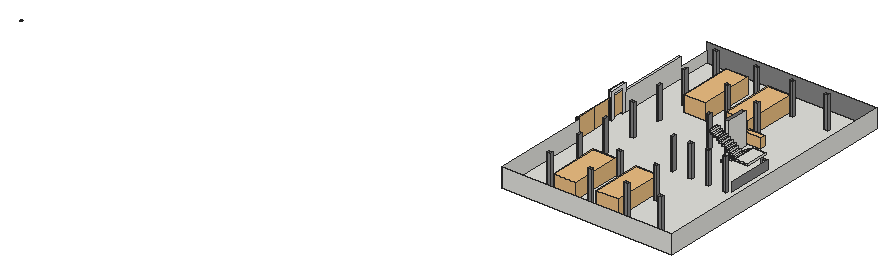
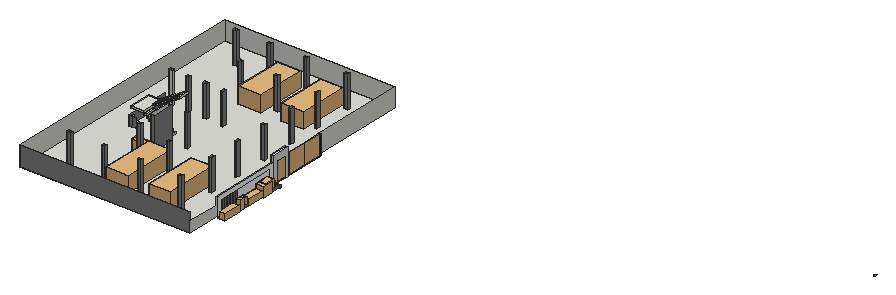
# SketchUp Ruby script. Lengths in inches.
U = 1.inch
M = Sketchup.active_model
def pt(a) = Geom::Point3d.new(a.map { |v| v * U })
def face(e, loops, mat)
  f = e.add_face(loops[0].map { |a| pt(a) })
  loops[1..].each { |l| e.add_face(l.map { |a| pt(a) }).erase! }
  f.material = f.back_material = mat if mat
  f
end
# faces: each face lists its corners as indices into pts; further lists are holes
def faces(e, pts, list, mat = nil) = list.each { |f| face(e, (f[0].is_a?(Array) ? f : [f]).map { |l| l.map { |i| pts[i] } }, mat) }
# xy, xz, yz: faces in a plane at the given z, y or x. An outline is a flat list of corners, or four numbers for a rectangle; further outlines are holes
def ring(l) = l.size == 4 ? [[l[0], l[1]], [l[2], l[1]], [l[2], l[3]], [l[0], l[3]]] : l.each_slice(2).to_a
def flat(e, list, mat, &to3) = list.each { |f| face(e, (f[0].is_a?(Array) ? f : [f]).map { |l| ring(l).map { |u, v| to3.(u, v) } }, mat) }
def xy(e, z, list, mat = nil) = flat(e, list, mat) { |x, y| [x, y, z] }
def xz(e, y, list, mat = nil) = flat(e, list, mat) { |x, z| [x, y, z] }
def yz(e, x, list, mat = nil) = flat(e, list, mat) { |y, z| [x, y, z] }
def lines(e, pts, list) = list.each { |a, b| e.add_line(pt(pts[a]), pt(pts[b])) }
# prism: a flat outline (further loops are holes) pulled along v
def prism(e, loops, v, mat = nil)
  f = face(e, loops, mat); d = Geom::Vector3d.new(v.map { |x| x * U })
  f.pushpull(f.normal.samedirection?(d) ? d.length : -d.length)
end
def box(e, o, s, mat = nil) = prism(e, [[o, [o[0] + s[0], o[1], o[2]], [o[0] + s[0], o[1] + s[1], o[2]], [o[0], o[1] + s[1], o[2]]]], [0, 0, s[2]], mat)
def at(x, y, z, deg = 0) = Geom::Transformation.translation(pt([x, y, z])) * Geom::Transformation.rotation(ORIGIN, Z_AXIS, deg.degrees)
def axes(o, x, y, z) = Geom::Transformation.new([*x, 0, *y, 0, *z, 0, *pt(o).to_a, 1])
def part(name) = M.definitions.add(name)
# library, detail: a bought-in or finely detailed component or shape, given as its bounding box
def library(name, o, s) = part(name).tap { |d| box(d.entities, o, s) }
def detail(e, o, s) = box(e.add_group.entities, o, s)
def put(e, d, t, mat = nil) = e.add_instance(d, t).tap { |i| i.material = mat if mat }
def group(e, t, mat = nil) = e.add_group.tap { |g| g.transformation = t; g.material = mat if mat }.entities
root = M.entities
M.materials.add("Bricks Weathered E01 100cm\#1").color = [154, 112, 93]
M.materials.add("Marble White 602 38.29cm").color = [255, 255, 255]
M.materials.add("Metal Black").color = [38, 38, 38]
M.materials.add("Mud Stones 01 100cm").color = [155, 124, 86]
M.materials.add("Paint Brown Gloss 1.5cm").color = [255, 255, 255]
M.materials.add("Wall Paint Bumpy 01 Gray 100cm").color = [135, 135, 135]
M.materials.add("Wood Planks C01 100cm\#1").color = [136, 107, 89]
M.materials.add("[Polished Concrete Old]").color = [229, 229, 229]
c1 = library("Comptonia peregrina 005",[-33.17,-28.03,-1.38],[76.14,61.63,51.11])
c2 = library("Potted Plant 02",[-16.98,-19.78,0],[30.04,38.68,37.52])
c3 = library("bike",[-29.48,-10.91,0],[58.96,21.79,36.68])
c4 = part("Rectangular post")
xy(c4.entities,0,[[0,0,2.7,4.37]])
xy(c4.entities,59.3,[[0,0,2.7,4.37]])
xz(c4.entities,0,[[0,0,2.7,59.3]])
xz(c4.entities,4.37,[[0,0,2.7,59.3]],"Wood Planks C01 100cm\#1")
yz(c4.entities,0,[[0,0,4.37,59.3]],"Wood Planks C01 100cm\#1")
yz(c4.entities,2.7,[[0,0,4.37,59.3]])
c5 = library("Group\#43",[0,0,0],[42,3,72])
c6 = library("Group\#38",[0.25,0,0],[71.75,3,72.2])
c7 = library("Group\#39",[0.25,0,0],[71.75,3,72.2])
c8 = part("Stair tread \#1")
box(c8.entities,[0,0,0],[10,39,7])
c9 = part("Stair tread")
box(c9.entities,[0,0,0],[10,39,7])
c10 = part("Group\#13")
box(c10.entities,[100,0,63],[49,84,7])
put(c10.entities,c8,at(50,45,28))
put(c10.entities,c8,at(20,45,7))
put(c10.entities,c8,at(90,45,56))
put(c10.entities,c8,at(70,45,42))
put(c10.entities,c8,at(40,45,21))
put(c10.entities,c8,at(60,45,35))
put(c10.entities,c8,at(10,45,0))
put(c10.entities,c8,at(30,45,14))
put(c10.entities,c8,at(80,45,49))
put(c10.entities,c9,at(90,0,70))
put(c10.entities,c9,at(10,0,126))
put(c10.entities,c9,at(60,0,91))
put(c10.entities,c9,at(30,0,112))
put(c10.entities,c9,at(50,0,98))
put(c10.entities,c9,at(70,0,84))
put(c10.entities,c9,at(80,0,77))
put(c10.entities,c9,at(40,0,105))
put(c10.entities,c9,at(0,0,133))
put(c10.entities,c9,at(20,0,119))
c11 = library("Car 038",[-41.0625,-100.42,-1.26],[82.125,200.85,59.95])
c12 = library("Group\#48",[0,0,0],[3.9375,4.89,0.01])
c13 = library("Group1671\#3",[0,0,0],[3.9375,4.89,0.39])
c14 = library("Group1672\#2",[0,0,0],[3.9375,4.89,0.39])
c15 = library("Car 033",[-43.24,-98.19,-1.29],[86.48,201.64,57.79])
c16 = library("Dalea purpurea 001",[-8.36,-8.34,-0.5],[17.08,16.6,23.28])
c17 = library("Car 026",[-43.02,-94.05,-1.1],[86.04,187.94,58.68])
c18 = library("Sedum Plant 66-24",[-7.97,-7.95,0.04],[16.42,16.31,19.57])
xy(root,0,[[[1741.02,413.67,2384.52,413.67,2384.52,1382.67,1741.02,1382.67,1741.02,1000.17,1729.02,1000.17,1729.02,778.17,1741.02,778.17],[2132.52,980.67,2146.52,1061.67],[1843.02,1286.67,1857.02,1295.67],[1843.02,500.67,1857.02,509.67],[2262.52,806.67,2276.52,815.67],[1843.02,641.67,1852.02,655.67],[1843.02,763.67,1852.02,777.67],[1843.02,1018.67,1852.02,1032.67],[1843.02,1140.67,1852.02,1154.67],[2066.52,806.67,2075.52,820.67],[2135.52,500.67,2149.52,509.67],[1997.02,638.67,2011.02,647.67],[2132.52,806.67,2146.52,815.67],[2066.52,975.67,2075.52,989.67],[1843.02,893.67,1857.02,902.67],[2132.52,1118.67,2146.52,1127.67],[1997.02,1148.67,2011.02,1157.67],[1997.02,1286.67,2011.02,1295.67],[1997.02,500.67,2011.02,509.67],[2262.52,500.67,2276.52,509.67],[2198.52,806.67,2212.52,815.67],[2262.52,1286.67,2276.52,1295.67],[2135.52,638.67,2149.52,647.67],[2132.52,1286.67,2146.52,1295.67]],[1843.02,500.67,1857.02,509.67],[1997.02,500.67,2011.02,509.67],[2135.52,500.67,2149.52,509.67],[2262.52,500.67,2276.52,509.67],
  [2132.52,989.67,2146.52,1061.67],[1843.02,1286.67,1857.02,1295.67],[1997.02,1286.67,2011.02,1295.67],[2132.52,1286.67,2146.52,1295.67],[2262.52,1286.67,2276.52,1295.67]])
xy(root,0,[[1709.32,1005.17,1733.02,1005.17,1733.02,1014.17,1740.02,1014.17,1740.02,1248.68,1733.02,1248.68,1733.02,1257.65,1709.32,1257.65]],"Mud Stones 01 100cm")
xy(root,0,[[1704.32,1000.17,1733.02,1001.07]],"Paint Brown Gloss 1.5cm")
xz(root,413.67,[[1741.02,0,2384.52,72]])
xz(root,500.67,[[1843.02,0,1857.02,120],[1997.02,0,2011.02,120],[2135.52,0,2149.52,120],[2262.52,0,2276.52,120]],"Wall Paint Bumpy 01 Gray 100cm")
xz(root,509.67,[[1843.02,0,1857.02,120],[1997.02,0,2011.02,120],[2135.52,0,2149.52,120],[2262.52,0,2276.52,120]],"Wall Paint Bumpy 01 Gray 100cm")
xz(root,638.67,[[1997.02,0,2011.02,120],[2135.52,0,2149.52,120]],"Wall Paint Bumpy 01 Gray 100cm")
xz(root,641.67,[[1843.02,0,1852.02,120]],"Wall Paint Bumpy 01 Gray 100cm")
xz(root,647.67,[[1997.02,0,2011.02,120],[2135.52,0,2149.52,120]],"Wall Paint Bumpy 01 Gray 100cm")
xz(root,655.67,[[1843.02,0,1852.02,120]],"Wall Paint Bumpy 01 Gray 100cm")
xz(root,763.67,[[1843.02,0,1852.02,120]],"Wall Paint Bumpy 01 Gray 100cm")
xz(root,777.67,[[1843.02,0,1852.02,120]],"Wall Paint Bumpy 01 Gray 100cm")
xz(root,778.17,[[1729.02,0,1741.02,72]])
xz(root,806.67,[[2066.52,0,2075.52,120],[2132.52,0,2146.52,120],[2198.52,0,2212.52,120],[2262.52,0,2276.52,120]],"Wall Paint Bumpy 01 Gray 100cm")
xz(root,815.67,[[2262.52,0,2276.52,120]])
xz(root,815.67,[[2132.52,0,2146.52,120],[2198.52,0,2212.52,120]],"Wall Paint Bumpy 01 Gray 100cm")
xz(root,820.67,[[2066.52,0,2075.52,120]],"Wall Paint Bumpy 01 Gray 100cm")
xz(root,893.67,[[1843.02,0,1857.02,120]],"Wall Paint Bumpy 01 Gray 100cm")
xz(root,902.67,[[1843.02,0,1857.02,120]],"Wall Paint Bumpy 01 Gray 100cm")
xz(root,975.67,[[2066.52,0,2075.52,120]],"Wall Paint Bumpy 01 Gray 100cm")
xz(root,980.67,[[2132.52,0,2146.52,120],[2276.52,0,2287.52,36]])
xz(root,989.67,[[2066.52,0,2075.52,120],[2262.52,0,2276.52,36],[2276.52,0,2288.52,36]],"Wall Paint Bumpy 01 Gray 100cm")
xz(root,1000.17,[[1723.05,0,1729.02,0.9,1729.02,0],[1729.02,0,1733.02,0.9],[1733.02,0,1741.02,72]])
xz(root,1000.17,[[1704.32,-2.82,1723.05,0,1704.32,0]],"Paint Brown Gloss 1.5cm")
xz(root,1001.07,[[1704.32,0,1733.02,9.5]],"Bricks Weathered E01 100cm\#1")
xz(root,1005.17,[[1709.32,0,1733.02,9.5]],"Bricks Weathered E01 100cm\#1")
xz(root,1014.17,[[1733.02,0,1740.02,58.01]])
xz(root,1018.67,[[1843.02,0,1852.02,120]],"Wall Paint Bumpy 01 Gray 100cm")
xz(root,1032.67,[[1843.02,0,1852.02,120]],"Wall Paint Bumpy 01 Gray 100cm")
xz(root,1061.67,[[2132.52,0,2146.52,120]],"Wall Paint Bumpy 01 Gray 100cm")
xz(root,1118.67,[[2132.52,0,2146.52,120]],"Wall Paint Bumpy 01 Gray 100cm")
xz(root,1127.67,[[2132.52,0,2146.52,120]],"Wall Paint Bumpy 01 Gray 100cm")
xz(root,1140.67,[[1843.02,0,1852.02,120]],"Wall Paint Bumpy 01 Gray 100cm")
xz(root,1148.67,[[1997.02,0,2011.02,120]],"Wall Paint Bumpy 01 Gray 100cm")
xz(root,1154.67,[[1843.02,0,1852.02,120]],"Wall Paint Bumpy 01 Gray 100cm")
xz(root,1157.67,[[1997.02,0,2011.02,120]],"Wall Paint Bumpy 01 Gray 100cm")
xz(root,1248.68,[[1733.02,0,1740.02,58.01]])
xz(root,1257.65,[[1709.32,0,1733.02,9.5]],"Bricks Weathered E01 100cm\#1")
xz(root,1286.67,[[1843.02,0,1857.02,120],[1997.02,0,2011.02,120],[2132.52,0,2146.52,120],[2262.52,0,2276.52,120]],"Wall Paint Bumpy 01 Gray 100cm")
xz(root,1295.67,[[1843.02,0,1857.02,120],[1997.02,0,2011.02,120],[2132.52,0,2146.52,120],[2262.52,0,2276.52,120]],"Wall Paint Bumpy 01 Gray 100cm")
xz(root,1382.67,[[1741.02,0,2384.52,72]],"Wall Paint Bumpy 01 Gray 100cm")
yz(root,1709.32,[[1005.17,0,1257.65,9.5]],"Bricks Weathered E01 100cm\#1")
yz(root,1729.02,[[778.97,0,1000.17,0.9]])
yz(root,1733.02,[[1000.17,0,1000.17,72,1262.67,72,1262.67,9.5,1257.65,9.5,1257.65,0,1248.68,0,1248.68,58.01,1014.17,58.01,1014.17,0,1005.17,0,1005.17,9.5,1001.07,9.5,1001.07,0]],"Paint Brown Gloss 1.5cm")
yz(root,1740.02,[[1014.17,0,1248.68,58.01]],"Marble White 602 38.29cm")
yz(root,1741.02,[[413.67,0,778.17,72],[1000.17,0,1382.67,0,1382.67,40.2,1262.67,40.2,1262.67,72,1000.17,72]])
yz(root,1843.02,[[500.67,0,509.67,120],[641.67,0,655.67,120],[763.67,0,777.67,120],[893.67,0,902.67,120],[1018.67,0,1032.67,120],
  [1140.67,0,1154.67,120],[1286.67,0,1295.67,120]],"Wall Paint Bumpy 01 Gray 100cm")
yz(root,1852.02,[[641.67,0,655.67,120],[763.67,0,777.67,120],[1018.67,0,1032.67,120],[1140.67,0,1154.67,120]],"Wall Paint Bumpy 01 Gray 100cm")
yz(root,1857.02,[[500.67,0,509.67,120],[893.67,0,902.67,120],[1286.67,0,1295.67,120]],"Wall Paint Bumpy 01 Gray 100cm")
yz(root,1997.02,[[500.67,0,509.67,120],[638.67,0,647.67,120],[1148.67,0,1157.67,120],[1286.67,0,1295.67,120]],"Wall Paint Bumpy 01 Gray 100cm")
yz(root,2011.02,[[500.67,0,509.67,120],[638.67,0,647.67,120],[1148.67,0,1157.67,120],[1286.67,0,1295.67,120]],"Wall Paint Bumpy 01 Gray 100cm")
yz(root,2066.52,[[806.67,0,820.67,120],[975.67,0,989.67,120]],"Wall Paint Bumpy 01 Gray 100cm")
yz(root,2075.52,[[806.67,0,820.67,120],[975.67,0,989.67,120]],"Wall Paint Bumpy 01 Gray 100cm")
yz(root,2132.52,[[806.67,0,815.67,120],[980.67,0,1061.67,120],[1118.67,0,1127.67,120],[1286.67,0,1295.67,120]],"Wall Paint Bumpy 01 Gray 100cm")
yz(root,2135.52,[[500.67,0,509.67,120],[638.67,0,647.67,120]],"Wall Paint Bumpy 01 Gray 100cm")
yz(root,2146.52,[[980.67,0,1061.67,120]])
yz(root,2146.52,[[806.67,0,815.67,120],[1118.67,0,1127.67,120],[1286.67,0,1295.67,120]],"Wall Paint Bumpy 01 Gray 100cm")
yz(root,2149.52,[[500.67,0,509.67,120],[638.67,0,647.67,120]],"Wall Paint Bumpy 01 Gray 100cm")
yz(root,2198.52,[[806.67,0,815.67,120]],"Wall Paint Bumpy 01 Gray 100cm")
yz(root,2212.52,[[806.67,0,815.67,120]],"Wall Paint Bumpy 01 Gray 100cm")
yz(root,2262.52,[[806.67,0,815.67,120]])
yz(root,2262.52,[[500.67,0,509.67,120],[1286.67,0,1295.67,120]],"Wall Paint Bumpy 01 Gray 100cm")
yz(root,2276.52,[[500.67,0,509.67,120],[806.67,0,815.67,120],[1286.67,0,1295.67,120]],"Wall Paint Bumpy 01 Gray 100cm")
yz(root,2288.52,[[819.67,0,989.67,36]],"Wall Paint Bumpy 01 Gray 100cm")
yz(root,2384.52,[[413.67,0,1382.67,72]])
p = [[2287.52,896.67,0],[2287.52,980.67,0],[2262.52,819.67,0],[2262.52,819.67,36],[2276.52,819.67,0],[2276.52,819.67,36]]
lines(root,p,[[0,1],[2,3],[4,5]])
put(root,c1,axes([1720.96,1102.63,-0.76],[0.35093,0,0],[0,1.23621,0],[0,0,0.45]))
put(root,c1,axes([1720.96,1220.98,-0.76],[0.35093,0,0],[0,1.10376,0],[0,0,0.45]))
put(root,c2,at(1721.91,1060.25,-0.83))
put(root,c3,at(2162.09,1086.83,0))
put(root,c4,at(1734.95,1233.17,0))
g1 = group(root,at(1741.02,778.17,0,90),"Wall Paint Bumpy 01 Gray 100cm")
put(g1,c5,at(168,5.5,3))
put(g1,c6,at(78,5.5,2.8))
g2 = group(g1,at(150,4,-3),"Metal Black")
box(g2,[0,0,3],[6,6,75])
put(g1,c7,axes([78,5.5,2.8],[-1,0,0],[0,1,0],[0,0,1]))
g3 = group(g1,at(0,4,-3),"Metal Black")
box(g3,[0,0,3],[6,6,75])
g4 = group(g1,at(156,0,3),"[Polished Concrete Old]")
xy(g4,-3,[[0,0,12,12],[54,0,66,12]])
xy(g4,73,[[12,6,54,12]])
xy(g4,84,[[12,0,54,6]])
xy(g4,96,[[0,0,66,12]])
xz(g4,0,[[0,-3,12,-3,12,84,54,84,54,-3,66,-3,66,96,0,96]])
xz(g4,6,[[12,73,54,84]])
xz(g4,12,[[0,-3,0,96,66,96,66,-3,54,-3,54,73,12,73,12,-3]])
yz(g4,0,[[0,-3,12,96]])
yz(g4,12,[[0,-3,12,-3,12,73,6,73,6,84,0,84]])
yz(g4,54,[[0,-3,0,84,6,84,6,73,12,73,12,-3]])
yz(g4,66,[[0,-3,12,96]])
put(root,c10,axes([2138.52,896.67,0],[1,0,0],[0,1,0],[0,0,0.9]))
put(root,c11,at(1916.46,1208.28,1.26))
put(root,c12,at(-1.18,313.15,0))
put(root,c13,at(-1.18,313.15,0))
put(root,c14,at(-1.18,313.15,0))
put(root,c15,at(2079.24,1202.24,1.29))
put(root,c16,axes([1717.66,1176.25,0.76],[1,0,0],[0,1,0],[0,0,1.53]))
put(root,c17,at(1913.82,589.9,1.1,180))
put(root,c17,at(2076.62,589.9,1.1,180))
put(root,c18,at(1724.99,1030.7,-0.04))
put(root,c4,at(1734.95,1220.17,0))
put(root,c4,at(1734.95,1207.17,0))
put(root,c4,at(1734.95,1194.17,0))
put(root,c4,at(1734.95,1181.17,0))
put(root,c4,at(1734.95,1168.17,0))
put(root,c2,at(1727.27,1044.38,0))
put(root,c18,at(1729.06,1013.08,0))
put(root,c18,axes([1723.87,1155.25,-0.02],[1,0,0],[0,1.18,0],[0,0,1.44]))
